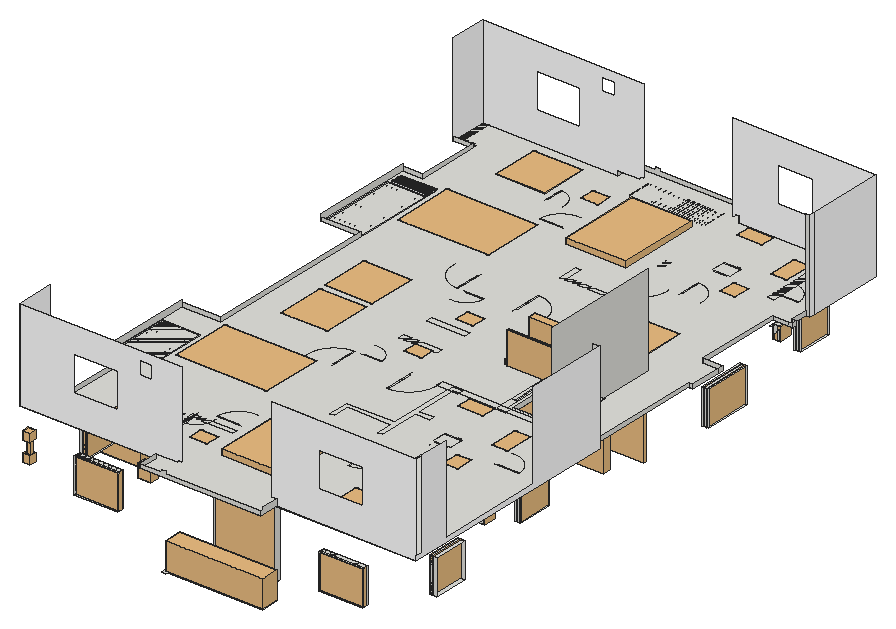
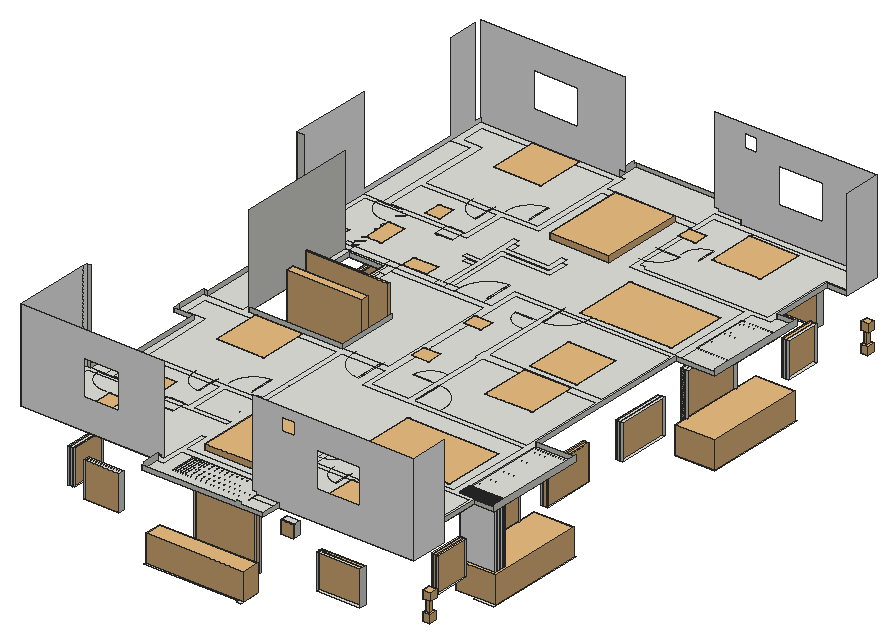
# SketchUp Ruby script. Lengths in inches.
U = 1.inch
M = Sketchup.active_model
def pt(a) = Geom::Point3d.new(a.map { |v| v * U })
def face(e, loops, mat)
  f = e.add_face(loops[0].map { |a| pt(a) })
  loops[1..].each { |l| e.add_face(l.map { |a| pt(a) }).erase! }
  f.material = f.back_material = mat if mat
  f
end
# faces: each face lists its corners as indices into pts; further lists are holes
def faces(e, pts, list, mat = nil) = list.each { |f| face(e, (f[0].is_a?(Array) ? f : [f]).map { |l| l.map { |i| pts[i] } }, mat) }
# xy, xz, yz: faces in a plane at the given z, y or x. An outline is a flat list of corners, or four numbers for a rectangle; further outlines are holes
def ring(l) = l.size == 4 ? [[l[0], l[1]], [l[2], l[1]], [l[2], l[3]], [l[0], l[3]]] : l.each_slice(2).to_a
def flat(e, list, mat, &to3) = list.each { |f| face(e, (f[0].is_a?(Array) ? f : [f]).map { |l| ring(l).map { |u, v| to3.(u, v) } }, mat) }
def xy(e, z, list, mat = nil) = flat(e, list, mat) { |x, y| [x, y, z] }
def xz(e, y, list, mat = nil) = flat(e, list, mat) { |x, z| [x, y, z] }
def yz(e, x, list, mat = nil) = flat(e, list, mat) { |y, z| [x, y, z] }
def lines(e, pts, list) = list.each { |a, b| e.add_line(pt(pts[a]), pt(pts[b])) }
# prism: a flat outline (further loops are holes) pulled along v
def prism(e, loops, v, mat = nil)
  f = face(e, loops, mat); d = Geom::Vector3d.new(v.map { |x| x * U })
  f.pushpull(f.normal.samedirection?(d) ? d.length : -d.length)
end
def box(e, o, s, mat = nil) = prism(e, [[o, [o[0] + s[0], o[1], o[2]], [o[0] + s[0], o[1] + s[1], o[2]], [o[0], o[1] + s[1], o[2]]]], [0, 0, s[2]], mat)
def at(x, y, z, deg = 0) = Geom::Transformation.translation(pt([x, y, z])) * Geom::Transformation.rotation(ORIGIN, Z_AXIS, deg.degrees)
def axes(o, x, y, z) = Geom::Transformation.new([*x, 0, *y, 0, *z, 0, *pt(o).to_a, 1])
def part(name) = M.definitions.add(name)
# library, detail: a bought-in or finely detailed component or shape, given as its bounding box
def library(name, o, s) = part(name).tap { |d| box(d.entities, o, s) }
def detail(e, o, s) = box(e.add_group.entities, o, s)
def put(e, d, t, mat = nil) = e.add_instance(d, t).tap { |i| i.material = mat if mat }
def group(e, t, mat = nil) = e.add_group.tap { |g| g.transformation = t; g.material = mat if mat }.entities
root = M.entities
M.materials.add("T8500 Silicone plaster D1 27.81cm").color = [255, 255, 255]
M.materials.add("Wintan - wpa36452 29.79cm").color = [255, 255, 255]
c1 = library("Group\#18",[0,0,0],[54.77,134.11,36.98])
c2 = library("Group\#21",[0,0,0],[134.45,23.44,36.98])
c3 = part("Rectangular column")
box(c3.entities,[0,16,0],[27,1,119.8])
box(c3.entities,[0,3.56,0],[27,1,120])
box(c3.entities,[0,1.78,0],[27,1,120])
box(c3.entities,[0,14.22,0],[27,1,119.8])
box(c3.entities,[0,5.33,0],[27,1,120])
box(c3.entities,[0,7.11,0],[27,1,120])
box(c3.entities,[0,10.67,0],[27,1,120.2])
box(c3.entities,[0,12.44,0],[27,1,119.8])
box(c3.entities,[0,0,0],[27,1,120])
xy(c3.entities,0,[[0,8.89,27,9.89]])
xy(c3.entities,120,[[0,8.89,27,9.89]])
xz(c3.entities,8.89,[[0,0,27,120]])
xz(c3.entities,9.89,[[0,0,27,120]])
yz(c3.entities,0,[[8.89,0,9.89,120]],"Wintan - wpa36452 29.79cm")
yz(c3.entities,27,[[8.89,0,9.89,120]])
c4 = library("Window Crafter Sliding",[0,-0.55,0],[84,4.49,96])
c5 = library("Group\#17",[0,0,0],[54.54,138.15,36.98])
c6 = library("Group\#23",[0,0,0],[133.24,24.34,36.98])
c7 = library("Door 243 053",[-21.6,-2.79,-0.07],[43.2,5.58,82.64])
c8 = library("Group\#6",[0,0,0],[112.45,3.15,94.27])
c9 = library("Group\#11",[0,0,0],[103.79,11.15,157.27])
c10 = library("Window Crafter Sliding 6",[0,-0.55,0],[72,4.49,48])
c11 = library("Window Crafter Sliding 2",[0,-0.55,0],[48,4.49,48])
c12 = library("Window Crafter Sliding 5",[0,-0.55,0],[66,4.49,48])
c13 = library("Window Crafter Sliding 3",[0,-0.55,0],[60,4.49,48])
c14 = library("Spot Light\#1",[-5.1,-5.1,-11.05],[10.2,10.2,11.05])
c15 = library("Lamp Wall Outdoor 94-02",[-1.89,-4.65,-3.17],[3.78,4.65,6.35])
c16 = library("Group\#12",[0,0,0],[113.66,3.15,100.57])
c17 = library("Window Crafter Awning 2",[0,-9.5,0],[17.5,11.27,18])
c18 = library("Tlon Light 650 Ceiling 152 007",[-12.8,-12.8,-3.78],[25.6,25.6,3.58])
c19 = part("Square rail bar")
box(c19.entities,[0,0,-1],[51.7,1,1])
c20 = part("Group\#20")
xy(c20.entities,0,[[0,0,51.7,106.6]])
xy(c20.entities,1,[[0,0,51.7,107.6]])
xz(c20.entities,0,[[0,0,51.7,1]])
xz(c20.entities,107.6,[[0,0,51.7,1]])
yz(c20.entities,0,[[0,0,107.6,1]])
yz(c20.entities,51.7,[[0,0,107.6,1]])
put(c20.entities,c19,at(0,106.6,0))
put(c20.entities,c19,at(0,0,0))
put(c20.entities,c19,at(0,103.05,0))
put(c20.entities,c19,at(0,99.49,0))
put(c20.entities,c19,at(0,95.94,0))
put(c20.entities,c19,at(0,92.39,0))
put(c20.entities,c19,at(0,88.83,0))
put(c20.entities,c19,at(0,85.28,0))
put(c20.entities,c19,at(0,81.73,0))
put(c20.entities,c19,at(0,78.17,0))
put(c20.entities,c19,at(0,74.62,0))
put(c20.entities,c19,at(0,71.07,0))
put(c20.entities,c19,at(0,67.51,0))
put(c20.entities,c19,at(0,63.96,0))
put(c20.entities,c19,at(0,60.41,0))
put(c20.entities,c19,at(0,56.85,0))
put(c20.entities,c19,at(0,53.3,0))
put(c20.entities,c19,at(0,49.75,0))
put(c20.entities,c19,at(0,46.19,0))
put(c20.entities,c19,at(0,42.64,0))
put(c20.entities,c19,at(0,39.09,0))
put(c20.entities,c19,at(0,35.53,0))
put(c20.entities,c19,at(0,31.98,0))
put(c20.entities,c19,at(0,28.43,0))
put(c20.entities,c19,at(0,24.875,0))
put(c20.entities,c19,at(0,21.32,0))
put(c20.entities,c19,at(0,17.77,0))
put(c20.entities,c19,at(0,14.21,0))
put(c20.entities,c19,at(0,10.66,0))
put(c20.entities,c19,at(0,7.11,0))
put(c20.entities,c19,at(0,3.55,0))
put(c20.entities,c19,at(0,0,0))
c21 = library("A$C403C54AD\#3",[0,0,-0.17],[8.08,5.86,0.57])
c22 = library("TARJA2\#3",[-2.49,-4.93,0],[8.71,4.91,0.01])
c23 = part("A$C42203764\#3")
put(c23.entities,c22,axes([263.32,520.21,0],[105.57605,0,0],[0,105.57605,0],[0,0,105.57605]))
c24 = library("A$C038F079D\#3",[0,0,0],[750,440,0.01])
c25 = library("A$C00C51FE0\#3",[0,0,0],[20,24.125,0.01])
c26 = library("A$C20C229D7\#3",[0,576,0],[24,24,0.01])
c27 = part("A$C659B0DF6\#3")
p = [[21.05,606.07,0],[21.05,607.55,0],[17.35,607.55,0],[17.35,606.07,0],[24,604.22,0],[0,604.22,0],
  [24,606.07,0],[0,606.07,0],[20.625,583.91,0],[20.625,585.72,0],[3.375,583.91,0],[3.375,585.72,0],
  [0,585.72,0],[24,585.72,0]]
lines(c27.entities,p,[[0,1],[2,3],[1,2],[4,5],[6,7],[8,9],[10,11],[10,8],[12,7],[13,6],[13,12]])
c28 = library("A$C4DC51D13\#3",[-0.71,0,0],[4438.2,2996.1875,0.01])
c29 = library("A$C52B64FF5\#3",[0,0,0],[6.95,7.1875,0.01])
c30 = part("*U13\#3")
p = [[0,0,0],[0,24,0],[-1.75,24,0],[-1.75,0,0],[-1.57,23.95,0],[-3.13,23.79,0],
  [-4.68,23.54,0],[-6.21,23.18,0],[-7.71,22.73,0],[-9.18,22.17,0],[-10.61,21.52,0],[-12,20.78,0],
  [-13.33,19.96,0],[-14.61,19.04,0],[-15.82,18.04,0],[-16.97,16.97,0],[-18.04,15.82,0],[-19.04,14.61,0],
  [-19.96,13.33,0],[-20.78,12,0],[-21.52,10.61,0],[-22.17,9.18,0],[-22.73,7.71,0],[-23.18,6.21,0],
  [-23.54,4.68,0],[-23.79,3.13,0],[-23.95,1.57,0],[-24,0,0],[0,-4,0],[-24,-4,0]]
lines(c30.entities,p,[[0,1],[1,2],[2,3],[3,0],[1,4],[4,5],[5,6],[6,7],[7,8],[8,9],[9,10],[10,11],
  [11,12],[12,13],[13,14],[14,15],[15,16],[16,17],[17,18],[18,19],[19,20],[20,21],[21,22],[22,23],
  [23,24],[24,25],[25,26],[26,27],[0,28],[27,29]])
c31 = part("*U14\#3")
p = [[0,0,0],[0,24,0],[1.75,24,0],[1.75,0,0],[24,0,0],[23.95,1.51,0],
  [23.8125,3.01,0],[23.57,4.5,0],[23.25,5.97,0],[22.83,7.42,0],[22.31,8.83,0],[21.72,10.22,0],
  [21.03,11.5625,0],[20.26,12.86,0],[19.42,14.11,0],[18.49,15.3,0],[17.5,16.43,0],[16.43,17.5,0],
  [15.3,18.49,0],[14.11,19.42,0],[12.86,20.26,0],[11.5625,21.03,0],[10.22,21.72,0],[8.83,22.31,0],
  [7.42,22.83,0],[5.97,23.25,0],[4.5,23.57,0],[3.01,23.8125,0],[1.51,23.95,0],[0,-4,0],
  [24,-4,0]]
lines(c31.entities,p,[[0,1],[1,2],[2,3],[3,0],[4,5],[5,6],[6,7],[7,8],[8,9],[9,10],[10,11],[11,12],
  [12,13],[13,14],[14,15],[15,16],[16,17],[17,18],[18,19],[19,20],[20,21],[21,22],[22,23],[23,24],
  [24,25],[25,26],[26,27],[27,28],[28,1],[0,29],[4,30]])
c32 = part("*U15\#3")
p = [[0,0,0],[0,30,0],[-1.75,30,0],[-1.75,0,0],[-1.96,29.9375,0],[-3.92,29.74,0],
  [-5.85,29.42,0],[-7.76,28.98,0],[-9.64,28.41,0],[-11.48,27.72,0],[-13.27,26.91,0],[-15,25.98,0],
  [-16.67,24.94,0],[-18.26,23.8,0],[-19.78,22.56,0],[-21.21,21.21,0],[-22.56,19.78,0],[-23.8,18.26,0],
  [-24.94,16.67,0],[-25.98,15,0],[-26.91,13.27,0],[-27.72,11.48,0],[-28.41,9.64,0],[-28.98,7.76,0],
  [-29.42,5.85,0],[-29.74,3.92,0],[-29.9375,1.96,0],[-30,0,0],[0,-4,0],[-30,-4,0]]
lines(c32.entities,p,[[0,1],[1,2],[2,3],[3,0],[1,4],[4,5],[5,6],[6,7],[7,8],[8,9],[9,10],[10,11],
  [11,12],[12,13],[13,14],[14,15],[15,16],[16,17],[17,18],[18,19],[19,20],[20,21],[21,22],[22,23],
  [23,24],[24,25],[25,26],[26,27],[0,28],[27,29]])
c33 = part("*U12\#3")
p = [[0,0,0],[0,-30,0],[-1.75,-30,0],[-1.75,0,0],[-30,0,0],[-29.94,-1.88,0],
  [-29.76,-3.76,0],[-29.47,-5.62,0],[-29.06,-7.46,0],[-28.53,-9.27,0],[-27.89,-11.04,0],[-27.14,-12.77,0],
  [-26.29,-14.45,0],[-25.33,-16.07,0],[-24.27,-17.63,0],[-23.12,-19.12,0],[-21.87,-20.54,0],[-20.54,-21.87,0],
  [-19.12,-23.12,0],[-17.63,-24.27,0],[-16.07,-25.33,0],[-14.45,-26.29,0],[-12.77,-27.14,0],[-11.04,-27.89,0],
  [-9.27,-28.53,0],[-7.46,-29.06,0],[-5.62,-29.47,0],[-3.76,-29.76,0],[-1.88,-29.94,0],[0,4,0],
  [-30,4,0]]
lines(c33.entities,p,[[0,1],[1,2],[2,3],[3,0],[4,5],[5,6],[6,7],[7,8],[8,9],[9,10],[10,11],[11,12],
  [12,13],[13,14],[14,15],[15,16],[16,17],[17,18],[18,19],[19,20],[20,21],[21,22],[22,23],[23,24],
  [24,25],[25,26],[26,27],[27,28],[28,1],[0,29],[4,30]])
c34 = part("*U9\#3")
p = [[0,0,0],[0,36,0],[-1.75,36,0],[-1.75,0,0],[-2.35,35.92,0],[-4.7,35.69,0],
  [-7.02,35.31,0],[-9.32,34.77,0],[-11.57,34.09,0],[-13.78,33.26,0],[-15.92,32.29,0],[-18,31.18,0],
  [-20,29.93,0],[-21.92,28.5625,0],[-23.74,27.07,0],[-25.46,25.46,0],[-27.07,23.74,0],[-28.5625,21.92,0],
  [-29.93,20,0],[-31.18,18,0],[-32.29,15.92,0],[-33.26,13.78,0],[-34.09,11.57,0],[-34.77,9.32,0],
  [-35.31,7.02,0],[-35.69,4.7,0],[-35.92,2.35,0],[-36,0,0],[0,-4,0],[-36,-4,0]]
lines(c34.entities,p,[[0,1],[1,2],[2,3],[3,0],[1,4],[4,5],[5,6],[6,7],[7,8],[8,9],[9,10],[10,11],
  [11,12],[12,13],[13,14],[14,15],[15,16],[16,17],[17,18],[18,19],[19,20],[20,21],[21,22],[22,23],
  [23,24],[24,25],[25,26],[26,27],[0,28],[27,29]])
c35 = part("*U8\#3")
p = [[0,0,0],[0,-36,0],[-1.75,-36,0],[-1.75,0,0],[-36,0,0],[-35.93,-2.26,0],
  [-35.72,-4.51,0],[-35.36,-6.75,0],[-34.87,-8.95,0],[-34.24,-11.125,0],[-33.47,-13.25,0],[-32.57,-15.33,0],
  [-31.55,-17.34,0],[-30.4,-19.29,0],[-29.125,-21.16,0],[-27.74,-22.95,0],[-26.24,-24.64,0],[-24.64,-26.24,0],
  [-22.95,-27.74,0],[-21.16,-29.125,0],[-19.29,-30.4,0],[-17.34,-31.55,0],[-15.33,-32.57,0],[-13.25,-33.47,0],
  [-11.125,-34.24,0],[-8.95,-34.87,0],[-6.75,-35.36,0],[-4.51,-35.72,0],[-2.26,-35.93,0],[0,4,0],
  [-36,4,0]]
lines(c35.entities,p,[[0,1],[1,2],[2,3],[3,0],[4,5],[5,6],[6,7],[7,8],[8,9],[9,10],[10,11],[11,12],
  [12,13],[13,14],[14,15],[15,16],[16,17],[17,18],[18,19],[19,20],[20,21],[21,22],[22,23],[23,24],
  [24,25],[25,26],[26,27],[27,28],[28,1],[0,29],[4,30]])
c36 = part("*U7\#3")
p = [[0,0,0],[0,24,0],[1.75,24,0],[1.75,0,0],[24,0,0],[23.95,1.51,0],
  [23.8125,3.01,0],[23.57,4.5,0],[23.25,5.97,0],[22.83,7.42,0],[22.31,8.83,0],[21.72,10.22,0],
  [21.03,11.5625,0],[20.26,12.86,0],[19.42,14.11,0],[18.49,15.3,0],[17.5,16.43,0],[16.43,17.5,0],
  [15.3,18.49,0],[14.11,19.42,0],[12.86,20.26,0],[11.5625,21.03,0],[10.22,21.72,0],[8.83,22.31,0],
  [7.42,22.83,0],[5.97,23.25,0],[4.5,23.57,0],[3.01,23.8125,0],[1.51,23.95,0],[0,-4,0],
  [24,-4,0]]
lines(c36.entities,p,[[0,1],[1,2],[2,3],[3,0],[4,5],[5,6],[6,7],[7,8],[8,9],[9,10],[10,11],[11,12],
  [12,13],[13,14],[14,15],[15,16],[16,17],[17,18],[18,19],[19,20],[20,21],[21,22],[22,23],[23,24],
  [24,25],[25,26],[26,27],[27,28],[28,1],[0,29],[4,30]])
c37 = part("*U6\#3")
p = [[0,0,0],[0,-24,0],[1.75,-24,0],[1.75,0,0],[1.51,-23.95,0],[3.01,-23.8125,0],
  [4.5,-23.57,0],[5.97,-23.25,0],[7.42,-22.83,0],[8.83,-22.31,0],[10.22,-21.72,0],[11.5625,-21.03,0],
  [12.86,-20.26,0],[14.11,-19.42,0],[15.3,-18.49,0],[16.43,-17.5,0],[17.5,-16.43,0],[18.49,-15.3,0],
  [19.42,-14.11,0],[20.26,-12.86,0],[21.03,-11.5625,0],[21.72,-10.22,0],[22.31,-8.83,0],[22.83,-7.42,0],
  [23.25,-5.97,0],[23.57,-4.5,0],[23.8125,-3.01,0],[23.95,-1.51,0],[24,0,0],[0,4,0],
  [24,4,0]]
lines(c37.entities,p,[[0,1],[1,2],[2,3],[3,0],[1,4],[4,5],[5,6],[6,7],[7,8],[8,9],[9,10],[10,11],
  [11,12],[12,13],[13,14],[14,15],[15,16],[16,17],[17,18],[18,19],[19,20],[20,21],[21,22],[22,23],
  [23,24],[24,25],[25,26],[26,27],[27,28],[0,29],[28,30]])
c38 = part("*U5\#3")
p = [[0,0,0],[0,-28,0],[1.75,-28,0],[1.75,0,0],[1.76,-27.94,0],[3.51,-27.78,0],
  [5.25,-27.5,0],[6.96,-27.12,0],[8.65,-26.63,0],[10.31,-26.03,0],[11.92,-25.34,0],[13.49,-24.54,0],
  [15,-23.64,0],[16.46,-22.65,0],[17.85,-21.57,0],[19.17,-20.41,0],[20.41,-19.17,0],[21.57,-17.85,0],
  [22.65,-16.46,0],[23.64,-15,0],[24.54,-13.49,0],[25.34,-11.92,0],[26.03,-10.31,0],[26.63,-8.65,0],
  [27.12,-6.96,0],[27.5,-5.25,0],[27.78,-3.51,0],[27.94,-1.76,0],[28,0,0],[0,4,0],
  [28,4,0]]
lines(c38.entities,p,[[0,1],[1,2],[2,3],[3,0],[1,4],[4,5],[5,6],[6,7],[7,8],[8,9],[9,10],[10,11],
  [11,12],[12,13],[13,14],[14,15],[15,16],[16,17],[17,18],[18,19],[19,20],[20,21],[21,22],[22,23],
  [23,24],[24,25],[25,26],[26,27],[27,28],[0,29],[28,30]])
c39 = part("*U4\#3")
p = [[0,0,0],[0,28,0],[1.75,28,0],[1.75,0,0],[28,0,0],[27.94,1.76,0],
  [27.78,3.51,0],[27.5,5.25,0],[27.12,6.96,0],[26.63,8.65,0],[26.03,10.31,0],[25.34,11.92,0],
  [24.54,13.49,0],[23.64,15,0],[22.65,16.46,0],[21.57,17.85,0],[20.41,19.17,0],[19.17,20.41,0],
  [17.85,21.57,0],[16.46,22.65,0],[15,23.64,0],[13.49,24.54,0],[11.92,25.34,0],[10.31,26.03,0],
  [8.65,26.63,0],[6.96,27.12,0],[5.25,27.5,0],[3.51,27.78,0],[1.76,27.94,0],[0,-4,0],
  [28,-4,0]]
lines(c39.entities,p,[[0,1],[1,2],[2,3],[3,0],[4,5],[5,6],[6,7],[7,8],[8,9],[9,10],[10,11],[11,12],
  [12,13],[13,14],[14,15],[15,16],[16,17],[17,18],[18,19],[19,20],[20,21],[21,22],[22,23],[23,24],
  [24,25],[25,26],[26,27],[27,28],[28,1],[0,29],[4,30]])
c40 = part("*U3\#3")
p = [[0,0,0],[0,30,0],[1.75,30,0],[1.75,0,0],[30,0,0],[29.94,1.88,0],
  [29.76,3.76,0],[29.47,5.62,0],[29.06,7.46,0],[28.53,9.27,0],[27.89,11.04,0],[27.14,12.77,0],
  [26.29,14.45,0],[25.33,16.07,0],[24.27,17.63,0],[23.12,19.12,0],[21.87,20.54,0],[20.54,21.87,0],
  [19.12,23.12,0],[17.63,24.27,0],[16.07,25.33,0],[14.45,26.29,0],[12.77,27.14,0],[11.04,27.89,0],
  [9.27,28.53,0],[7.46,29.06,0],[5.62,29.47,0],[3.76,29.76,0],[1.88,29.94,0],[0,-4,0],
  [30,-4,0]]
lines(c40.entities,p,[[0,1],[1,2],[2,3],[3,0],[4,5],[5,6],[6,7],[7,8],[8,9],[9,10],[10,11],[11,12],
  [12,13],[13,14],[14,15],[15,16],[16,17],[17,18],[18,19],[19,20],[20,21],[21,22],[22,23],[23,24],
  [24,25],[25,26],[26,27],[27,28],[28,1],[0,29],[4,30]])
c41 = part("*U2\#3")
p = [[0,0,0],[0,-32,0],[1.75,-32,0],[1.75,0,0],[2.01,-31.9375,0],[4.01,-31.75,0],
  [6,-31.43,0],[7.96,-30.99,0],[9.89,-30.43,0],[11.78,-29.75,0],[13.625,-28.95,0],[15.42,-28.04,0],
  [17.15,-27.02,0],[18.81,-25.89,0],[20.4,-24.66,0],[21.91,-23.33,0],[23.33,-21.91,0],[24.66,-20.4,0],
  [25.89,-18.81,0],[27.02,-17.15,0],[28.04,-15.42,0],[28.95,-13.625,0],[29.75,-11.78,0],[30.43,-9.89,0],
  [30.99,-7.96,0],[31.43,-6,0],[31.75,-4.01,0],[31.9375,-2.01,0],[32,0,0],[0,4,0],
  [32,4,0]]
lines(c41.entities,p,[[0,1],[1,2],[2,3],[3,0],[1,4],[4,5],[5,6],[6,7],[7,8],[8,9],[9,10],[10,11],
  [11,12],[12,13],[13,14],[14,15],[15,16],[16,17],[17,18],[18,19],[19,20],[20,21],[21,22],[22,23],
  [23,24],[24,25],[25,26],[26,27],[27,28],[0,29],[28,30]])
c42 = part("Commercial Building Flr Plans.dwg\#3")
xy(c42.entities,0,[[722.01,373.53,728.01,373.53,728.01,396.03,788.01,396.03,788.01,373.53,794.01,373.53,794.01,430.53,814.01,430.53,814.01,436.53,794.01,436.53,794.01,493.53,923.01,493.53,923.01,487.53,932.01,487.53,932.01,493.53,918.01,493.53,918.01,502.53,868.01,502.53,868.01,493.53,854.01,493.53,854.01,502.53,773.01,502.53,773.01,493.53,788.01,493.53,788.01,502.53,802.01,502.53,802.01,493.53,788.01,493.53,788.01,402.03,722.01,402.03],[854.01,493.53,868.01,502.53],[918.01,493.53,932.01,502.53],[854.01,502.53,863.01,520.53],[[863.01,502.53,923.01,574.53],[867.01,506.53,915.01,570.53]],
  [923.01,502.53,932.01,502.53,932.01,583.53,932.01,574.53,923.01,574.53],[854.01,520.53,859.01,520.53,859.01,538.53,858.01,538.53,858.01,556.53,854.01,556.53],[859.01,520.53,860.01,538.53],[860.01,520.53,863.01,520.53,863.01,556.53,859.01,556.53,859.01,538.53,860.01,538.53],[858.01,538.53,859.01,556.53],
  [854.01,556.53,863.01,574.53],[854.01,574.53,868.01,583.53],[918.01,574.53,932.01,583.53]])
xz(c42.entities,506.53,[[867.01,-6,915.01,0]])
xz(c42.entities,570.53,[[867.01,-6,915.01,0]])
yz(c42.entities,867.01,[[506.53,-6,570.53,0]])
yz(c42.entities,915.01,[[506.53,-6,570.53,0]])
# 5414 loose lines left out
put(c42.entities,c21,axes([684.95,938.32,0.02],[0,-14.03023,0],[14.03023,0,0],[0,0,14.03023]))
put(c42.entities,c21,axes([684.95,346.29,0.02],[0,-14.03023,0],[14.03023,0,0],[0,0,14.03023]))
put(c42.entities,c23,axes([900.04,908.53,0],[0,0.04349,0],[0.04349,0,0],[0,0,0.04349]))
put(c42.entities,c23,axes([900.04,428.53,0],[0,0.04349,0],[0.04349,0,0],[0,0,0.04349]))
put(c42.entities,c24,axes([819.23,471.91,0],[0.04545,0,0],[0,0.04545,0],[0,0,0.04545]))
put(c42.entities,c24,axes([819.23,951.91,0],[0.04545,0,0],[0,0.04545,0],[0,0,0.04545]))
put(c42.entities,c25,axes([722.01,550.53,0],[0,-1,0],[-1,0,0],[0,0,1]))
put(c42.entities,c25,at(660.51,238.53,0,90))
put(c42.entities,c25,at(722.01,619.53,0,90))
put(c42.entities,c25,at(660.51,911.53,0,90))
put(c42.entities,c25,at(901.51,868.5,0,180))
put(c42.entities,c25,at(904.51,388.5,0,180))
put(c42.entities,c26,at(942.55,371.21,0))
put(c42.entities,c26,at(945.55,-108.79,0))
put(c42.entities,c27,at(845.01,-189.39,0))
put(c42.entities,c27,at(845.01,290.61,0))
put(c42.entities,c28,axes([512.64,369.84,0],[0.02827,0,0],[0,0.02827,0],[0,0,0.02827]))
put(c42.entities,c28,axes([512.64,750.84,0],[0.02827,0,0],[0,0.02827,0],[0,0,0.02827]))
put(c42.entities,c29,axes([533.03,959.68,0],[0,-9.39007,0],[9.39007,0,0],[0,0,9.39007]))
put(c42.entities,c29,axes([841.85,744,0],[9.39007,0,0],[0,-9.39007,0],[0,0,9.39007]))
put(c42.entities,c29,axes([844.85,264,0],[9.39007,0,0],[0,-9.39007,0],[0,0,9.39007]))
put(c42.entities,c29,axes([541.85,657,0],[9.39007,0,0],[0,-9.39007,0],[0,0,9.39007]))
put(c42.entities,c29,axes([541.85,513.06,0],[9.39007,0,0],[0,9.39007,0],[0,0,9.39007]))
put(c42.entities,c29,axes([533.03,275.68,0],[0,-9.39007,0],[9.39007,0,0],[0,0,9.39007]))
put(c42.entities,c30,at(669.51,496.53,0,-90))
put(c42.entities,c31,at(669.51,673.53,0,-90))
put(c42.entities,c32,at(932.01,397.53,0,-90))
put(c42.entities,c32,at(932.01,877.53,0,-90))
put(c42.entities,c33,at(660.51,292.53,0,-90))
put(c42.entities,c33,at(660.51,847.03,0,-90))
put(c42.entities,c34,at(657.51,460.53,0))
put(c42.entities,c35,at(657.51,709.53,0))
put(c42.entities,c36,at(609.51,886.53,0))
put(c42.entities,c37,at(609.51,283.53,0))
put(c42.entities,c38,axes([734.01,493.53,0],[1.39286,0,0],[0,1.39286,0],[0,0,1.39286]))
put(c42.entities,c39,axes([734.01,676.53,0],[1.39286,0,0],[0,1.39286,0],[0,0,1.39286]))
put(c42.entities,c40,at(854.01,334.53,0))
put(c42.entities,c40,at(851.01,814.53,0))
put(c42.entities,c41,at(807.51,328.53,0))
put(c42.entities,c41,at(804.51,808.53,0))
xy(root,129,[[2005.02,473.67,2011.02,473.67,2011.02,476.67,2141.52,476.67,2141.52,500.67,2135.52,500.67,2135.52,482.67,2011.02,482.67,2011.02,500.67,2005.02,500.67],[2031.27,530.62,2115.27,539.67],[1789.02,637.17,1816.02,637.17,1816.02,643.17,1795.02,643.17,1795.02,772.17,1843.02,772.17,1843.02,778.17,1789.02,778.17],[1843.02,673.67,1852.02,757.67],[1789.02,1018.17,1843.02,1018.17,1843.02,1024.17,1795.02,1024.17,1795.02,1148.67,1816.02,1148.67,1816.02,1159.17,1789.02,1159.17],
  [1843.02,1046.67,1852.02,1130.67],[2031.27,1256.67,2115.27,1265.67],[2005.02,1295.67,2011.02,1295.67,2011.02,1313.67,2135.52,1313.67,2135.52,1295.67,2141.52,1295.67,2141.52,1319.67,2011.02,1319.67,2011.02,1322.67,2005.02,1322.67]])
xy(root,162,[[1863.02,500.67,1923.02,509.67],[2199.52,500.67,2259.52,509.67],[1816.02,569.57,1825.02,617.57],[2297.52,569.57,2306.52,617.57],[2267.52,752.67,2276.52,800.67],
  [1843.02,797.67,1852.02,869.67],[1843.02,926.67,1852.02,998.67],[2294.52,1040.67,2303.52,1106.67],[1816.02,1172.67,1825.02,1220.67],[2267.52,1232.67,2276.52,1280.67],
  [1863.02,1286.67,1923.02,1295.67],[2195.52,1286.67,2243.52,1295.67]])
xy(root,210,[[1863.02,500.67,1923.02,509.67],[2199.52,500.67,2259.52,509.67],[1816.02,569.57,1825.02,617.57],[2297.52,569.57,2306.52,617.57],[1954.02,596.67,1978.02,602.67],
  [2005.02,605.67,2011.02,635.67],[2152.02,641.67,2184.02,647.67],[2198.52,641.67,2228.52,647.67],[2267.52,710.67,2276.52,740.67],[2267.52,752.67,2276.52,800.67],
  [1966.02,767.67,2002.02,773.67],[1843.02,797.67,1852.02,869.67],[2078.52,806.67,2117.52,815.67],[2008.02,809.67,2014.02,833.67],[1843.02,926.67,1852.02,998.67],
  [2008.02,962.67,2014.02,986.67],[2078.52,980.67,2117.52,989.67],[1966.02,1022.67,2002.02,1028.67],[2294.52,1040.67,2303.52,1106.67],[2149.02,1121.67,2181.02,1127.67],
  [2195.52,1121.67,2225.52,1127.67],[2005.02,1160.17,2011.02,1190.17],[1816.02,1172.67,1825.02,1220.67],[2267.52,1190.67,2276.52,1220.67],[1954.02,1193.67,1978.02,1199.67],
  [2267.52,1232.67,2276.52,1280.67],[1863.02,1286.67,1923.02,1295.67],[2195.52,1286.67,2243.52,1295.67]])
xy(root,216,[[1953.02,500.67,1970.52,509.67],[2297.52,649.73,2306.52,667.23],[2029.77,869.67,2047.27,878.67],[2029.77,917.67,2047.27,926.67],[2294.52,1162.17,2303.52,1179.67],
  [1953.02,1286.67,1970.52,1295.67]])
xy(root,225,[[2031.27,530.62,2115.27,539.67],[1843.02,673.67,1852.02,757.67],[1843.02,1046.67,1852.02,1130.67],[2031.27,1256.67,2115.27,1265.67]])
xy(root,234,[[1953.02,500.67,1970.52,509.67],[2297.52,649.73,2306.52,667.23],[2029.77,869.67,2047.27,878.67],[2029.77,917.67,2047.27,926.67],[2294.52,1162.17,2303.52,1179.67],
  [1953.02,1286.67,1970.52,1295.67]])
xy(root,246,[[[1975.05,473.67,1975.05,500.67,1789.02,500.67,1789.02,551.67,1816.02,551.67,1816.02,637.17,1789.02,637.17,1789.02,778.17,1843.02,778.17,1843.02,1018.17,1789.02,1018.17,1789.02,1159.17,1816.02,1159.17,1816.02,1244.67,1789.02,1244.67,1789.02,1295.67,1975.05,1295.67,1975.05,1322.67,2141.52,1322.67,2141.52,1295.67,2330.52,1295.67,2330.52,1181.67,2324.52,1181.67,2324.52,1157.7,2330.52,1157.7,2330.52,1151.7,2303.52,1151.7,2303.52,1031.67,2330.52,1031.67,2330.52,980.67,2324.52,980.67,2324.52,815.67,2333.52,815.67,2333.52,500.67,2141.52,500.67,2141.52,473.67],[2138.52,896.67,2267.52,980.67],[2211.52,819.67,2259.52,883.67]],[[1789.02,500.67,2011.02,500.67,2011.02,647.67,1852.02,647.67,1852.02,767.67,2072.52,767.67,2072.52,806.67,2132.52,806.67,2132.52,715.17,2066.52,715.17,2066.52,686.67,2072.52,686.67,2072.52,709.17,2132.52,709.17,2132.52,686.67,2138.52,686.67,2138.52,743.67,2158.52,743.67,2158.52,749.67,2138.52,749.67,2138.52,806.67,2324.52,806.67,2324.52,815.67,2276.52,815.67,2276.52,980.67,2330.52,980.67,2330.52,1031.67,2303.52,1031.67,2303.52,1151.7,2324.52,1151.7,2324.52,1157.7,2303.52,1157.7,2303.52,1181.67,2330.52,1181.67,2330.52,1295.67,2132.52,1295.67,2132.52,1223.67,2138.52,1223.67,2138.52,1286.67,2324.52,1286.67,2324.52,1187.67,2132.52,1187.67,2132.52,1181.67,2183.52,1181.67,2183.52,1127.67,2132.52,1127.67,2132.52,989.67,2072.52,989.67,2072.52,1028.67,1852.02,1028.67,1852.02,1148.67,2011.02,1148.67,2011.02,1256.67,2132.52,1256.67,2132.52,1265.67,2011.02,1265.67,2011.02,1295.67,1798.02,1295.67,1798.02,1286.67,1945.02,1286.67,1945.02,1193.67,2005.02,1193.67,2005.02,1157.67,1997.02,1157.67,1997.02,1154.67,1825.02,1154.67,1825.02,1253.67,1816.02,1253.67,1816.02,1148.67,1843.02,1148.67,1843.02,647.67,1816.02,647.67,1816.02,551.67,1789.02,551.67],[1852.02,773.67,1852.02,893.67,2014.02,893.67,2014.02,891.17,2017.02,891.17,2017.02,905.17,2014.02,905.17,2014.02,902.67,1852.02,902.67,1852.02,1022.67,2008.02,1022.67,2008.02,902.67,2014.02,902.67,2014.02,1022.67,2066.52,1022.67,2066.52,773.67,2014.02,773.67,2014.02,893.67,2008.02,893.67,2008.02,773.67],[2075.52,815.67,2267.52,980.67],[1798.02,509.67,1798.02,542.67,1825.02,542.67,1825.02,641.67,1997.02,641.67,1997.02,638.67,2005.02,638.67,2005.02,509.67],[2138.52,989.67,2138.52,1118.67,2146.52,1118.67,2146.52,1121.67,2294.52,1121.67,2294.52,1022.67,2321.52,1022.67,2321.52,989.67],[2189.52,1127.67,2294.52,1181.67],[1951.02,1199.67,2005.02,1286.67]],[[2135.52,500.67,2333.52,500.67,2333.52,551.67,2306.52,551.67,2306.52,701.67,2333.52,701.67,2333.52,806.67,2327.52,806.67,2327.52,707.67,2186.52,707.67,2186.52,647.67,2135.52,647.67,2135.52,539.67,2011.02,539.67,2011.02,530.62,2135.52,530.62],[2141.52,509.67,2141.52,641.67,2297.52,641.67,2297.52,542.67,2324.52,542.67,2324.52,509.67],[2192.52,647.67,2297.52,701.67]],[1945.02,509.67,1951.02,509.67,1951.02,596.67,2005.02,596.67,2005.02,602.67,1945.02,602.67],[2267.52,707.67,2276.52,806.67],
  [2324.52,806.67,2333.52,815.67],[2014.02,869.67,2066.52,878.67],[2014.02,917.67,2066.52,926.67],[2066.52,1081.17,2132.52,1081.17,2132.52,1087.17,2072.52,1087.17,2072.52,1109.67,2066.52,1109.67],[2132.52,1157.67,2138.52,1181.67],
  [2267.52,1187.67,2276.52,1286.67],[1789.02,1244.67,1816.02,1244.67,1816.02,1253.67,1798.02,1253.67,1798.02,1295.67,1789.02,1295.67]])
xz(root,473.67,[[1975.05,246,2141.52,246,2141.52,252,2011.02,252,2011.02,255,2005.02,255,2005.02,252,1975.05,252]])
xz(root,500.67,[[[1789.02,246,1975.05,246,1975.05,252,2005.02,252,2005.02,255,2011.02,255,2011.02,372,1789.02,372],[1863.02,288,1923.02,336],[1953.02,342,1970.52,360]],[[2141.52,246,2333.52,246,2333.52,372,2135.52,372,2135.52,255,2141.52,255],[2199.52,288,2259.52,336]]],"T8500 Silicone plaster D1 27.81cm")
xz(root,551.67,[[1789.02,246,1816.02,252]])
xz(root,569.57,[[1816.02,162,1825.02,210],[2297.52,162,2306.52,210]])
xz(root,617.57,[[1816.02,162,1825.02,210],[2297.52,162,2306.52,210]])
xz(root,637.17,[[1789.02,246,1816.02,252]])
xz(root,649.73,[[2297.52,216,2306.52,234]])
xz(root,667.23,[[2297.52,216,2306.52,234]])
xz(root,673.67,[[1843.02,129,1852.02,225]])
xz(root,752.67,[[2267.52,162,2276.52,210]])
xz(root,757.67,[[1843.02,129,1852.02,225]])
xz(root,778.17,[[1789.02,246,1843.02,252]])
xz(root,797.67,[[1843.02,162,1852.02,210]])
xz(root,800.67,[[2267.52,162,2276.52,210]])
xz(root,815.67,[[2324.52,246,2333.52,372]])
xz(root,869.67,[[1843.02,162,1852.02,210]])
xz(root,896.67,[[2138.52,246,2267.52,252]])
xz(root,926.67,[[1843.02,162,1852.02,210]])
xz(root,980.67,[[2138.52,246,2267.52,252],[2324.52,246,2330.52,252]])
xz(root,998.67,[[1843.02,162,1852.02,210]])
xz(root,1018.17,[[1789.02,246,1843.02,252]])
xz(root,1031.67,[[2303.52,246,2330.52,252]])
xz(root,1040.67,[[2294.52,162,2303.52,210]])
xz(root,1046.67,[[1843.02,129,1852.02,225]])
xz(root,1106.67,[[2294.52,162,2303.52,210]])
xz(root,1130.67,[[1843.02,129,1852.02,225]])
xz(root,1151.7,[[2303.52,246,2324.52,252],[2324.52,246,2330.52,252]])
xz(root,1157.7,[[2324.52,246,2330.52,252]])
xz(root,1159.17,[[1789.02,246,1816.02,252]])
xz(root,1162.17,[[2294.52,216,2303.52,234]])
xz(root,1172.67,[[1816.02,162,1825.02,210]])
xz(root,1179.67,[[2294.52,216,2303.52,234]])
xz(root,1181.67,[[2324.52,246,2330.52,372]])
xz(root,1220.67,[[1816.02,162,1825.02,210]])
xz(root,1232.67,[[2267.52,162,2276.52,210]])
xz(root,1244.67,[[1789.02,246,1816.02,252]])
xz(root,1280.67,[[2267.52,162,2276.52,210]])
xz(root,1295.67,[[[1789.02,246,1789.02,372,2011.02,372,2011.02,255,2005.02,255,2005.02,252,1975.05,252,1975.05,246],[1863.02,288,1923.02,336],[1953.02,342,1970.52,360]],[[2141.52,246,2141.52,255,2135.52,255,2135.52,252,2132.52,252,2132.52,372,2330.52,372,2330.52,246],[2195.52,288,2243.52,336]]],"T8500 Silicone plaster D1 27.81cm")
xz(root,1322.67,[[1975.05,246,1975.05,252,2005.02,252,2005.02,255,2011.02,255,2011.02,252,2141.52,252,2141.52,246]])
yz(root,1789.02,[[637.17,246,778.17,255],[1018.17,246,1159.17,255]])
yz(root,1789.02,[[500.67,246,551.67,372],[1244.67,246,1295.67,372]],"T8500 Silicone plaster D1 27.81cm")
yz(root,1816.02,[[551.67,246,637.17,252],[1159.17,246,1244.67,252]])
yz(root,1843.02,[[778.17,246,1018.17,252]])
yz(root,1863.02,[[500.67,162,509.67,210],[1286.67,162,1295.67,210]])
yz(root,1923.02,[[500.67,162,509.67,210],[1286.67,162,1295.67,210]])
yz(root,1953.02,[[500.67,216,509.67,234],[1286.67,216,1295.67,234]])
yz(root,1970.52,[[500.67,216,509.67,234],[1286.67,216,1295.67,234]])
yz(root,1975.05,[[473.67,246,500.67,252],[1295.67,246,1322.67,252]])
yz(root,2029.77,[[869.67,216,878.67,234],[917.67,216,926.67,234]])
yz(root,2031.27,[[530.62,129,539.67,225],[1256.67,129,1265.67,225]])
yz(root,2047.27,[[869.67,216,878.67,234],[917.67,216,926.67,234]])
yz(root,2115.27,[[530.62,129,539.67,225],[1256.67,129,1265.67,225]])
yz(root,2138.52,[[896.67,246,980.67,252]])
yz(root,2141.52,[[473.67,246,500.67,246,500.67,255,476.67,255,476.67,252,473.67,252],[1295.67,246,1322.67,246,1322.67,252,1319.67,252,1319.67,255,1295.67,255]])
yz(root,2195.52,[[1286.67,162,1295.67,210]])
yz(root,2199.52,[[500.67,162,509.67,210]])
yz(root,2243.52,[[1286.67,162,1295.67,210]])
yz(root,2259.52,[[500.67,162,509.67,210]])
yz(root,2267.52,[[896.67,246,896.67,252,815.67,252,815.67,372,980.67,372,980.67,246]])
yz(root,2303.52,[[1031.67,246,1151.7,252]])
yz(root,2324.52,[[815.67,246,980.67,252],[1157.7,246,1181.67,252]])
yz(root,2330.52,[[980.67,246,1022.67,252],[1022.67,246,1031.67,252],[1151.7,246,1157.7,252]])
yz(root,2330.52,[[1181.67,246,1187.67,372],[1187.67,246,1295.67,372]],"T8500 Silicone plaster D1 27.81cm")
yz(root,2333.52,[[500.67,246,815.67,246,815.67,372,701.67,372,701.67,252,551.67,252,551.67,372,509.67,372,509.67,252,500.67,252]],"T8500 Silicone plaster D1 27.81cm")
put(root,c1,at(1790.22,1019.37,128.41))
put(root,c2,at(2005.77,1293.7,128.98))
put(root,c3,axes([1795.02,1131.67,129],[1.77778,0,0],[0,1,0],[0,0,0.98781]),"Wintan - wpa36452 29.79cm")
put(root,c4,at(2031.27,533.26,129))
put(root,c4,at(1849.22,1046.67,129,90))
put(root,c4,at(2031.27,1259.48,129))
put(root,c4,at(1851.46,673.67,129,90))
put(root,c5,at(1790.45,638.6,129))
put(root,c6,at(2006.65,478.3,129))
put(root,c7,axes([2011.02,821.67,129.14],[0,-0.55585,0],[1.07698,0,0],[0,0,1.01843]))
put(root,c8,at(2152.15,978.1,132.3))
put(root,c9,at(2141.95,933.1,132.3))
put(root,c10,at(1844.98,998.67,162,-90))
put(root,c11,at(2270.52,1280.67,162,-90))
put(root,c11,at(1818.83,1220.67,162,-90))
put(root,c10,at(1847.52,869.67,162,-90))
put(root,c12,at(2300.72,1040.67,162,90))
put(root,c13,at(2199.52,503.48,162))
put(root,c11,at(1820.52,617.57,162,-90))
put(root,c13,at(1863.02,503.48,162))
put(root,c11,at(2270.52,800.67,162,-90))
put(root,c13,at(1863.02,1287.79,162))
put(root,c11,at(2297.52,617.57,162,-90))
put(root,c11,at(2243.52,1293.71,162,180))
put(root,c14,at(1784.03,1275.46,176.28))
put(root,c14,at(1784.03,522.625,176.28))
put(root,c15,axes([1787.14,1275.32,184.51],[0,-1,0],[1,0,0],[0,0,2.6448]))
put(root,c15,axes([1787.14,522.48,184.51],[0,-1,0],[1,0,0],[0,0,2.6448]))
put(root,c16,at(2141.95,896.1,189))
put(root,c14,axes([1783.68,1275.18,192.79],[1,0,0],[0,1,0],[0,0,-1]))
put(root,c14,axes([1783.68,522.34,192.79],[1,0,0],[0,1,0],[0,0,-1]))
put(root,c17,at(2029.77,924.9,216))
put(root,c17,at(2047.27,869.67,216,180))
put(root,c17,at(2296.3,1162.17,216,90))
put(root,c17,at(1970.52,1288.45,216,180))
put(root,c17,at(2299.3,649.73,216,90))
put(root,c17,at(1953.02,507.9,216))
put(root,c18,axes([2034,1282.86,243.8125],[0.44,0,0],[0,0.44,0],[0,0,0.44]))
put(root,c18,axes([2077.86,1282.86,243.8125],[0.44,0,0],[0,0.44,0],[0,0,0.44]))
put(root,c18,axes([1817.33,1094.72,244.24],[0.44,0,0],[0,0.44,0],[0,0,0.44]))
put(root,c18,axes([1817.33,1048.52,244.24],[0.44,0,0],[0,0.44,0],[0,0,0.44]))
put(root,c18,axes([1817.33,723.4375,244.24],[0.44,0,0],[0,0.44,0],[0,0,0.44]))
put(root,c18,axes([1817.33,677.24,244.24],[0.44,0,0],[0,0.44,0],[0,0,0.44]))
put(root,c20,axes([2011.02,1301.77,244.6],[0,-0.69826,0],[0.97119,0,0],[0,0,1]))
put(root,c20,at(1791.32,1022.61,245))
put(root,c20,axes([1791.32,664.54,245],[1,0,0],[0,0.72,0],[0,0,1]))
put(root,c42,at(1344.52,313.15,252))
